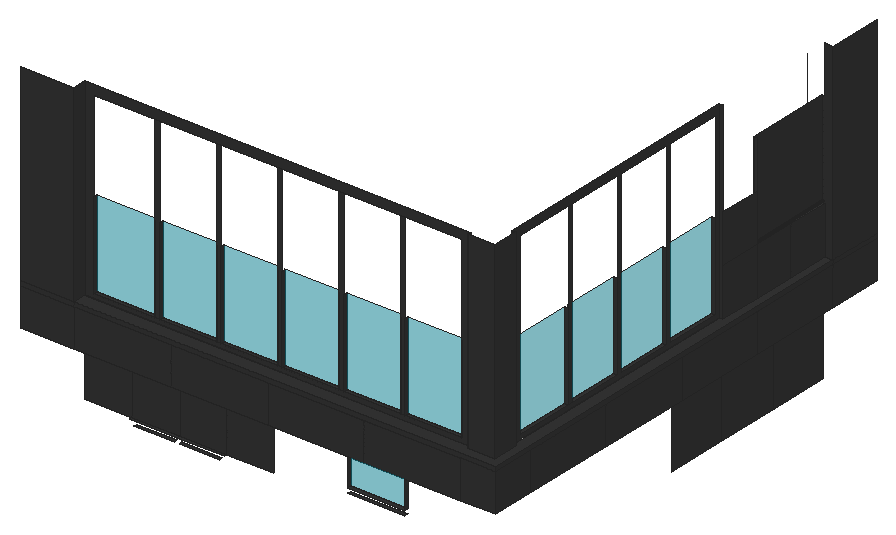
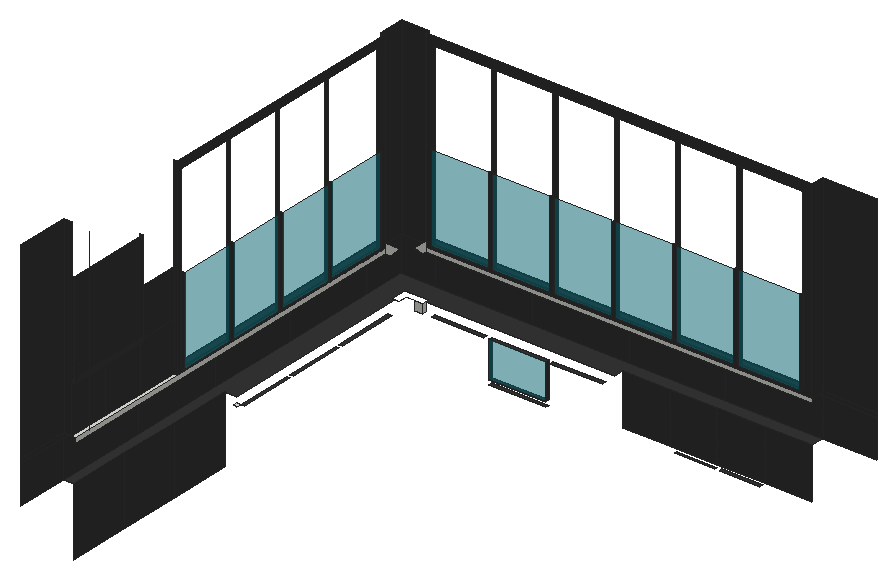
# SketchUp Ruby script. Lengths in inches.
U = 1.inch
M = Sketchup.active_model
def pt(a) = Geom::Point3d.new(a.map { |v| v * U })
def face(e, loops, mat)
  f = e.add_face(loops[0].map { |a| pt(a) })
  loops[1..].each { |l| e.add_face(l.map { |a| pt(a) }).erase! }
  f.material = f.back_material = mat if mat
  f
end
# faces: each face lists its corners as indices into pts; further lists are holes
def faces(e, pts, list, mat = nil) = list.each { |f| face(e, (f[0].is_a?(Array) ? f : [f]).map { |l| l.map { |i| pts[i] } }, mat) }
# xy, xz, yz: faces in a plane at the given z, y or x. An outline is a flat list of corners, or four numbers for a rectangle; further outlines are holes
def ring(l) = l.size == 4 ? [[l[0], l[1]], [l[2], l[1]], [l[2], l[3]], [l[0], l[3]]] : l.each_slice(2).to_a
def flat(e, list, mat, &to3) = list.each { |f| face(e, (f[0].is_a?(Array) ? f : [f]).map { |l| ring(l).map { |u, v| to3.(u, v) } }, mat) }
def xy(e, z, list, mat = nil) = flat(e, list, mat) { |x, y| [x, y, z] }
def xz(e, y, list, mat = nil) = flat(e, list, mat) { |x, z| [x, y, z] }
def yz(e, x, list, mat = nil) = flat(e, list, mat) { |y, z| [x, y, z] }
def lines(e, pts, list) = list.each { |a, b| e.add_line(pt(pts[a]), pt(pts[b])) }
# prism: a flat outline (further loops are holes) pulled along v
def prism(e, loops, v, mat = nil)
  f = face(e, loops, mat); d = Geom::Vector3d.new(v.map { |x| x * U })
  f.pushpull(f.normal.samedirection?(d) ? d.length : -d.length)
end
def box(e, o, s, mat = nil) = prism(e, [[o, [o[0] + s[0], o[1], o[2]], [o[0] + s[0], o[1] + s[1], o[2]], [o[0], o[1] + s[1], o[2]]]], [0, 0, s[2]], mat)
def at(x, y, z, deg = 0) = Geom::Transformation.translation(pt([x, y, z])) * Geom::Transformation.rotation(ORIGIN, Z_AXIS, deg.degrees)
def axes(o, x, y, z) = Geom::Transformation.new([*x, 0, *y, 0, *z, 0, *pt(o).to_a, 1])
def part(name) = M.definitions.add(name)
# library, detail: a bought-in or finely detailed component or shape, given as its bounding box
def library(name, o, s) = part(name).tap { |d| box(d.entities, o, s) }
def detail(e, o, s) = box(e.add_group.entities, o, s)
def put(e, d, t, mat = nil) = e.add_instance(d, t).tap { |i| i.material = mat if mat }
def group(e, t, mat = nil) = e.add_group.tap { |g| g.transformation = t; g.material = mat if mat }.entities
root = M.entities
M.materials.add("[0135_DarkGray]1").color = [53, 53, 53]
M.materials.add("[Translucent Glass Blue]1").color = [1, 149, 171]
M.materials["[Translucent Glass Blue]1"].alpha = 0.5
xy(root,197.67,[[554.94,728.6875,609.19,732.6875],[615.19,728.6875,669.44,732.6875]],"[0135_DarkGray]1")
xy(root,203.67,[[548.94,728.6875,612.19,732.6875],[612.19,728.6875,675.44,732.6875]],"[0135_DarkGray]1")
xy(root,204.96,[[827.03,745.6875,903.36,750.6875]],"[0135_DarkGray]1")
xy(root,211.2,[[827.03,745.6875,903.36,750.6875]],"[0135_DarkGray]1")
xy(root,259.5625,[[1018.69,1020.6875,1023.69,1026.6875]])
xy(root,259.5625,[[750.69,745.6875,821.03,750.6875],[827.03,745.6875,903.36,750.6875],[909.36,745.6875,979.69,750.6875],[1013.69,774.6875,1018.69,856.6875],[1013.69,862.6875,1018.69,938.6875],
  [1013.69,944.6875,1018.69,1020.6875]],"[0135_DarkGray]1")
xy(root,271.5625,[[485.69,714.6875,485.69,732.6875,738.69,732.6875,738.69,745.6875,991.69,745.6875,991.69,740.6875,1023.69,740.6875,1023.69,762.6875,1018.69,762.6875,1018.69,1026.6875,1035.69,1026.6875,1035.69,1278.6875,1049.69,1278.6875,1049.69,714.6875]],"[0135_DarkGray]1")
xy(root,328.25,[[1033.13,1108.6875,1038.13,1278.6875]])
xy(root,328.25,[[485.69,714.6875,1049.69,714.6875,1049.69,1278.6875,1038.13,1278.6875,1038.13,1108.6875,1033.13,1108.6875,1033.13,762.6875,1038.13,762.6875,1038.13,727.5625,1001.69,727.5625,1001.69,732.5625,485.69,732.5625]],"[0135_DarkGray]1")
xy(root,334.25,[[497.69,732.5625,579.69,737.5625],[585.69,732.5625,661.69,737.5625],[667.69,732.5625,743.69,737.5625],[749.69,732.5625,825.69,737.5625],[831.69,732.5625,907.69,737.5625],
  [913.69,732.5625,989.69,737.5625],[1028.13,774.6875,1033.13,856.6875],[1028.13,862.6875,1033.13,938.6875],[1028.13,944.6875,1033.13,1020.6875],[1028.13,1026.6875,1033.13,1102.6875]],"[0135_DarkGray]1")
xy(root,392.3125,[[1034.13,1165.35,1038.13,1222.02],[1034.13,1222.02,1038.13,1278.6875]],"[0135_DarkGray]1")
xy(root,393.26,[[1035.97,1165.35,1036.3125,1278.6875]],"[0135_DarkGray]1")
xy(root,395.86,[[1035.96,1165.35,1036.3,1278.6875]],"[0135_DarkGray]1")
xz(root,714.6875,[[413.69,271.5625,485.69,322.25],[485.69,271.5625,615.01,322.25],[615.01,271.5625,744.32,322.25],[744.32,271.5625,873.63,322.25],[873.63,271.5625,1002.94,322.25],
  [1002.94,271.5625,1049.69,322.25],[413.69,322.25,485.69,328.25],[485.69,322.25,1049.69,328.25],[413.69,328.25,485.69,584.5]],"[0135_DarkGray]1")
xz(root,727.5625,[[1001.69,328.25,1038.13,584.5]],"[0135_DarkGray]1")
xz(root,732.5625,[[485.69,322.25,1001.69,328.25]])
xz(root,732.5625,[[[485.69,328.25,1001.69,584.5],[497.69,334.25,989.69,572.5]],[579.69,334.25,585.69,572.5],[661.69,334.25,667.69,572.5],[743.69,334.25,749.69,572.5],[825.69,334.25,831.69,572.5],
  [907.69,334.25,913.69,572.5]],"[0135_DarkGray]1")
xz(root,732.6875,[[485.69,203.67,548.94,271.5625],[548.94,203.67,612.19,271.5625],[612.19,203.67,675.44,271.5625],[675.44,203.67,738.69,271.5625]],"[0135_DarkGray]1")
xz(root,737.5625,[[497.69,334.25,579.69,450.375],[585.69,334.25,661.69,450.375],[667.69,334.25,743.69,450.375],[749.69,334.25,825.69,450.375],[831.69,334.25,907.69,450.375],
  [913.69,334.25,989.69,450.375]],"[Translucent Glass Blue]1")
xz(root,750.6875,[[991.69,259.5625,1001.69,271.5625]])
xz(root,750.6875,[[827.03,211.2,903.36,259.5625]],"[Translucent Glass Blue]1")
xz(root,762.6875,[[1025.13,322.25,1033.13,322.25,1033.13,334.25,1013.69,334.25]])
xz(root,762.6875,[[1033.13,328.25,1038.13,584.5]],"[0135_DarkGray]1")
xz(root,774.6875,[[1028.13,334.25,1033.13,450.375]],"[0135_DarkGray]1")
xz(root,856.6875,[[1028.13,334.25,1033.13,450.375]],"[0135_DarkGray]1")
xz(root,862.6875,[[1028.13,334.25,1033.13,450.375]],"[0135_DarkGray]1")
xz(root,938.6875,[[1028.13,334.25,1033.13,450.375]],"[0135_DarkGray]1")
xz(root,944.6875,[[1028.13,334.25,1033.13,450.375]],"[0135_DarkGray]1")
xz(root,1020.6875,[[1028.13,334.25,1033.13,450.375]],"[0135_DarkGray]1")
xz(root,1026.6875,[[1028.13,334.25,1033.13,450.375]],"[0135_DarkGray]1")
xz(root,1102.6875,[[1028.13,334.25,1033.13,450.375]],"[0135_DarkGray]1")
xz(root,1108.6875,[[1033.13,328.25,1038.13,584.5]],"[0135_DarkGray]1")
xz(root,1165.35,[[[1034.13,392.3125,1038.13,520.4375],[1035.97,517.26,1036.3125,517.26,1036.64,517.35,1036.94,517.52,1037.18,517.77,1037.35,518.0625,1037.4375,518.4,1037.44,518.74,1037.34,519.07,1037.17,519.36,1036.93,519.61,1036.63,519.77,1036.3,519.86,1035.96,519.86,1035.625,519.77,1035.33,519.6,1035.09,519.35,1034.92,519.05,1034.83,518.72,1034.83,518.38,1034.93,518.05,1035.1,517.75,1035.34,517.51,1035.64,517.34],[1035.97,513.125,1036.3125,513.125,1036.64,513.22,1036.94,513.39,1037.18,513.63,1037.35,513.93,1037.4375,514.26,1037.44,514.6,1037.34,514.94,1037.17,515.23,1036.93,515.47,1036.63,515.64,1036.3,515.73,1035.96,515.73,1035.625,515.64,1035.33,515.46,1035.09,515.22,1034.92,514.92,1034.83,514.59,1034.83,514.25,1034.93,513.92,1035.1,513.62,1035.34,513.38,1035.64,513.21],[1035.97,508.99,1036.3125,508.99,1036.64,509.08,1036.94,509.26,1037.18,509.5,1037.35,509.8,1037.4375,510.13,1037.44,510.47,1037.34,510.8,1037.17,511.1,1036.93,511.34,1036.63,511.51,1036.3,511.6,1035.96,511.59,1035.625,511.5,1035.33,511.33,1035.09,511.09,1034.92,510.79,1034.83,510.46,1034.83,510.11,1034.93,509.78,1035.1,509.49,1035.34,509.25,1035.64,509.08],[1035.97,504.86,1036.3125,504.86,1036.64,504.95,1036.94,505.12,1037.18,505.37,1037.35,505.66,1037.4375,506,1037.44,506.34,1037.34,506.67,1037.17,506.96,1036.93,507.21,1036.63,507.375,1036.3,507.46,1035.96,507.46,1035.625,507.37,1035.33,507.2,1035.09,506.95,1034.92,506.65,1034.83,506.32,1034.83,505.98,1034.93,505.65,1035.1,505.35,1035.34,505.11,1035.64,504.94],[1035.97,500.72,1036.3125,500.73,1036.64,500.82,1036.94,500.99,1037.18,501.23,1037.35,501.53,1037.4375,501.86,1037.44,502.2,1037.34,502.54,1037.17,502.83,1036.93,503.07,1036.63,503.24,1036.3,503.33,1035.96,503.33,1035.625,503.24,1035.33,503.0625,1035.09,502.82,1034.92,502.52,1034.83,502.19,1034.83,501.85,1034.93,501.52,1035.1,501.22,1035.34,500.98,1035.64,500.8125],[1035.97,496.59,1036.3125,496.59,1036.64,496.68,1036.94,496.86,1037.18,497.1,1037.35,497.4,1037.4375,497.73,1037.44,498.07,1037.34,498.4,1037.17,498.7,1036.93,498.9375,1036.63,499.11,1036.3,499.2,1035.96,499.19,1035.625,499.1,1035.33,498.93,1035.09,498.6875,1034.92,498.39,1034.83,498.06,1034.83,497.71,1034.93,497.38,1035.1,497.09,1035.34,496.85,1035.64,496.68],[1035.97,492.46,1036.3125,492.46,1036.64,492.55,1036.94,492.72,1037.18,492.97,1037.35,493.26,1037.4375,493.6,1037.44,493.9375,1037.34,494.27,1037.17,494.5625,1036.93,494.81,1036.63,494.97,1036.3,495.0625,1035.96,495.06,1035.625,494.97,1035.33,494.8,1035.09,494.55,1034.92,494.25,1034.83,493.92,1034.83,493.58,1034.93,493.25,1035.1,492.95,1035.34,492.71,1035.64,492.54],[1035.97,488.32,1036.3125,488.33,1036.64,488.42,1036.94,488.59,1037.18,488.83,1037.35,489.13,1037.4375,489.46,1037.44,489.8,1037.34,490.14,1037.17,490.43,1036.93,490.67,1036.63,490.84,1036.3,490.93,1035.96,490.93,1035.625,490.84,1035.33,490.66,1035.09,490.42,1034.92,490.12,1034.83,489.79,1034.83,489.45,1034.93,489.12,1035.1,488.82,1035.34,488.58,1035.64,488.41],[1035.97,484.19,1036.3125,484.19,1036.64,484.28,1036.94,484.46,1037.18,484.7,1037.35,485,1037.4375,485.33,1037.44,485.67,1037.34,486,1037.17,486.3,1036.93,486.54,1036.63,486.71,1036.3,486.8,1035.96,486.79,1035.625,486.7,1035.33,486.53,1035.09,486.29,1034.92,485.99,1034.83,485.66,1034.83,485.3125,1034.93,484.98,1035.1,484.6875,1035.34,484.45,1035.64,484.28],[1035.97,480.06,1036.3125,480.06,1036.64,480.15,1036.94,480.32,1037.18,480.57,1037.35,480.86,1037.4375,481.2,1037.44,481.54,1037.34,481.87,1037.17,482.16,1036.93,482.41,1036.63,482.57,1036.3,482.66,1035.96,482.66,1035.625,482.57,1035.33,482.4,1035.09,482.15,1034.92,481.85,1034.83,481.52,1034.83,481.18,1034.93,480.85,1035.1,480.55,1035.34,480.3125,1035.64,480.14],[1035.97,475.92,1036.3125,475.93,1036.64,476.02,1036.94,476.1875,1037.18,476.43,1037.35,476.73,1037.4375,477.0625,1037.44,477.4,1037.34,477.74,1037.17,478.03,1036.93,478.27,1036.63,478.44,1036.3,478.53,1035.96,478.53,1035.625,478.4375,1035.33,478.26,1035.09,478.02,1034.92,477.72,1034.83,477.39,1034.83,477.05,1034.93,476.72,1035.1,476.42,1035.34,476.18,1035.64,476.01],[1035.97,471.79,1036.3125,471.79,1036.64,471.88,1036.94,472.06,1037.18,472.3,1037.35,472.6,1037.4375,472.93,1037.44,473.27,1037.34,473.6,1037.17,473.9,1036.93,474.14,1036.63,474.31,1036.3,474.4,1035.96,474.39,1035.625,474.3,1035.33,474.13,1035.09,473.89,1034.92,473.59,1034.83,473.26,1034.83,472.91,1034.93,472.58,1035.1,472.29,1035.34,472.05,1035.64,471.88],[1035.97,467.66,1036.3125,467.66,1036.64,467.75,1036.94,467.92,1037.18,468.17,1037.35,468.46,1037.4375,468.8,1037.44,469.14,1037.34,469.47,1037.17,469.76,1036.93,470.01,1036.63,470.17,1036.3,470.26,1035.96,470.26,1035.625,470.17,1035.33,470,1035.09,469.75,1034.92,469.45,1034.83,469.125,1034.83,468.78,1034.93,468.45,1035.1,468.15,1035.34,467.91,1035.64,467.74],[1035.97,463.52,1036.3125,463.53,1036.64,463.62,1036.94,463.79,1037.18,464.03,1037.35,464.33,1037.4375,464.66,1037.44,465,1037.34,465.34,1037.17,465.63,1036.93,465.87,1036.63,466.04,1036.3,466.13,1035.96,466.125,1035.625,466.04,1035.33,465.86,1035.09,465.62,1034.92,465.32,1034.83,464.99,1034.83,464.65,1034.93,464.32,1035.1,464.02,1035.34,463.78,1035.64,463.61],[1035.97,459.39,1036.3125,459.39,1036.64,459.48,1036.94,459.66,1037.18,459.9,1037.35,460.2,1037.4375,460.53,1037.44,460.87,1037.34,461.2,1037.17,461.5,1036.93,461.74,1036.63,461.91,1036.3,462,1035.96,461.99,1035.625,461.9,1035.33,461.73,1035.09,461.49,1034.92,461.1875,1034.83,460.86,1034.83,460.51,1034.93,460.18,1035.1,459.89,1035.34,459.65,1035.64,459.48],[1035.97,455.26,1036.3125,455.26,1036.64,455.35,1036.94,455.52,1037.18,455.77,1037.35,456.0625,1037.4375,456.4,1037.44,456.74,1037.34,457.07,1037.17,457.36,1036.93,457.61,1036.63,457.77,1036.3,457.86,1035.96,457.86,1035.625,457.77,1035.33,457.6,1035.09,457.35,1034.92,457.05,1034.83,456.72,1034.83,456.38,1034.93,456.05,1035.1,455.75,1035.34,455.51,1035.64,455.34],[1035.97,451.125,1036.3125,451.125,1036.64,451.22,1036.94,451.39,1037.18,451.63,1037.35,451.93,1037.4375,452.26,1037.44,452.6,1037.34,452.94,1037.17,453.23,1036.93,453.47,1036.63,453.64,1036.3,453.73,1035.96,453.73,1035.625,453.64,1035.33,453.46,1035.09,453.22,1034.92,452.92,1034.83,452.59,1034.83,452.25,1034.93,451.92,1035.1,451.62,1035.34,451.38,1035.64,451.21],[1035.97,446.99,1036.3125,446.99,1036.64,447.08,1036.94,447.26,1037.18,447.5,1037.35,447.8,1037.4375,448.13,1037.44,448.47,1037.34,448.8,1037.17,449.1,1036.93,449.34,1036.63,449.51,1036.3,449.6,1035.96,449.59,1035.625,449.5,1035.33,449.33,1035.09,449.09,1034.92,448.79,1034.83,448.46,1034.83,448.11,1034.93,447.78,1035.1,447.49,1035.34,447.25,1035.64,447.08],[1035.97,442.86,1036.3125,442.86,1036.64,442.95,1036.94,443.12,1037.18,443.37,1037.35,443.66,1037.4375,444,1037.44,444.34,1037.34,444.67,1037.17,444.96,1036.93,445.21,1036.63,445.375,1036.3,445.46,1035.96,445.46,1035.625,445.37,1035.33,445.2,1035.09,444.95,1034.92,444.65,1034.83,444.32,1034.83,443.98,1034.93,443.65,1035.1,443.35,1035.34,443.11,1035.64,442.94],[1035.97,438.72,1036.3125,438.73,1036.64,438.82,1036.94,438.99,1037.18,439.23,1037.35,439.53,1037.4375,439.86,1037.44,440.2,1037.34,440.54,1037.17,440.83,1036.93,441.07,1036.63,441.24,1036.3,441.33,1035.96,441.33,1035.625,441.24,1035.33,441.0625,1035.09,440.82,1034.92,440.52,1034.83,440.19,1034.83,439.85,1034.93,439.52,1035.1,439.22,1035.34,438.98,1035.64,438.8125],[1035.97,434.59,1036.3125,434.59,1036.64,434.68,1036.94,434.86,1037.18,435.1,1037.35,435.4,1037.4375,435.73,1037.44,436.07,1037.34,436.4,1037.17,436.7,1036.93,436.9375,1036.63,437.11,1036.3,437.2,1035.96,437.19,1035.625,437.1,1035.33,436.93,1035.09,436.6875,1034.92,436.39,1034.83,436.06,1034.83,435.71,1034.93,435.38,1035.1,435.09,1035.34,434.85,1035.64,434.68],[1035.97,430.46,1036.3125,430.46,1036.64,430.55,1036.94,430.72,1037.18,430.97,1037.35,431.26,1037.4375,431.6,1037.44,431.9375,1037.34,432.27,1037.17,432.5625,1036.93,432.81,1036.63,432.97,1036.3,433.0625,1035.96,433.06,1035.625,432.97,1035.33,432.8,1035.09,432.55,1034.92,432.25,1034.83,431.92,1034.83,431.58,1034.93,431.25,1035.1,430.95,1035.34,430.71,1035.64,430.54],[1035.97,426.32,1036.3125,426.33,1036.64,426.42,1036.94,426.59,1037.18,426.83,1037.35,427.13,1037.4375,427.46,1037.44,427.8,1037.34,428.14,1037.17,428.43,1036.93,428.67,1036.63,428.84,1036.3,428.93,1035.96,428.93,1035.625,428.84,1035.33,428.66,1035.09,428.42,1034.92,428.12,1034.83,427.79,1034.83,427.45,1034.93,427.12,1035.1,426.82,1035.34,426.58,1035.64,426.41],[1035.97,422.19,1036.3125,422.19,1036.64,422.28,1036.94,422.46,1037.18,422.7,1037.35,423,1037.4375,423.33,1037.44,423.67,1037.34,424,1037.17,424.3,1036.93,424.54,1036.63,424.71,1036.3,424.8,1035.96,424.79,1035.625,424.7,1035.33,424.53,1035.09,424.29,1034.92,423.99,1034.83,423.66,1034.83,423.3125,1034.93,422.98,1035.1,422.6875,1035.34,422.45,1035.64,422.28],[1035.97,418.06,1036.3125,418.06,1036.64,418.15,1036.94,418.32,1037.18,418.57,1037.35,418.86,1037.4375,419.2,1037.44,419.54,1037.34,419.87,1037.17,420.16,1036.93,420.41,1036.63,420.57,1036.3,420.66,1035.96,420.66,1035.625,420.57,1035.33,420.4,1035.09,420.15,1034.92,419.85,1034.83,419.52,1034.83,419.18,1034.93,418.85,1035.1,418.55,1035.34,418.3125,1035.64,418.14],[1035.97,413.92,1036.3125,413.93,1036.64,414.02,1036.94,414.1875,1037.18,414.43,1037.35,414.73,1037.4375,415.0625,1037.44,415.4,1037.34,415.74,1037.17,416.03,1036.93,416.27,1036.63,416.44,1036.3,416.53,1035.96,416.53,1035.625,416.4375,1035.33,416.26,1035.09,416.02,1034.92,415.72,1034.83,415.39,1034.83,415.05,1034.93,414.72,1035.1,414.42,1035.34,414.18,1035.64,414.01],[1035.97,409.79,1036.3125,409.79,1036.64,409.88,1036.94,410.06,1037.18,410.3,1037.35,410.6,1037.4375,410.93,1037.44,411.27,1037.34,411.6,1037.17,411.9,1036.93,412.14,1036.63,412.31,1036.3,412.4,1035.96,412.39,1035.625,412.3,1035.33,412.13,1035.09,411.89,1034.92,411.59,1034.83,411.26,1034.83,410.91,1034.93,410.58,1035.1,410.29,1035.34,410.05,1035.64,409.88],[1035.97,405.66,1036.3125,405.66,1036.64,405.75,1036.94,405.92,1037.18,406.17,1037.35,406.46,1037.4375,406.8,1037.44,407.14,1037.34,407.47,1037.17,407.76,1036.93,408.01,1036.63,408.17,1036.3,408.26,1035.96,408.26,1035.625,408.17,1035.33,408,1035.09,407.75,1034.92,407.45,1034.83,407.125,1034.83,406.78,1034.93,406.45,1035.1,406.15,1035.34,405.91,1035.64,405.74],[1035.97,401.52,1036.3125,401.53,1036.64,401.62,1036.94,401.79,1037.18,402.03,1037.35,402.33,1037.4375,402.66,1037.44,403,1037.34,403.34,1037.17,403.63,1036.93,403.87,1036.63,404.04,1036.3,404.13,1035.96,404.125,1035.625,404.04,1035.33,403.86,1035.09,403.62,1034.92,403.32,1034.83,402.99,1034.83,402.65,1034.93,402.32,1035.1,402.02,1035.34,401.78,1035.64,401.61],[1035.97,397.39,1036.3125,397.39,1036.64,397.48,1036.94,397.66,1037.18,397.9,1037.35,398.2,1037.4375,398.53,1037.44,398.87,1037.34,399.2,1037.17,399.5,1036.93,399.74,1036.63,399.91,1036.3,400,1035.96,399.99,1035.625,399.9,1035.33,399.73,1035.09,399.49,1034.92,399.1875,1034.83,398.86,1034.83,398.51,1034.93,398.18,1035.1,397.89,1035.34,397.65,1035.64,397.48],[1035.97,393.26,1036.3125,393.26,1036.64,393.35,1036.94,393.52,1037.18,393.77,1037.35,394.0625,1037.4375,394.4,1037.44,394.74,1037.34,395.07,1037.17,395.36,1036.93,395.61,1036.63,395.77,1036.3,395.86,1035.96,395.86,1035.625,395.77,1035.33,395.6,1035.09,395.35,1034.92,395.05,1034.83,394.72,1034.83,394.38,1034.93,394.05,1035.1,393.75,1035.34,393.51,1035.64,393.34]]],"[0135_DarkGray]1")
xz(root,1278.6875,[[[1038.13,328.25,1049.69,328.25,1049.69,584.5,1038.13,584.5,1038.13,520.4375,1034.13,520.4375,1034.13,392.3125,1038.13,392.3125],[1035.97,517.26,1035.64,517.34,1035.34,517.51,1035.1,517.75,1034.93,518.05,1034.83,518.38,1034.83,518.72,1034.92,519.05,1035.09,519.35,1035.33,519.6,1035.625,519.77,1035.96,519.86,1036.3,519.86,1036.63,519.77,1036.93,519.61,1037.17,519.36,1037.34,519.07,1037.44,518.74,1037.4375,518.4,1037.35,518.0625,1037.18,517.77,1036.94,517.52,1036.64,517.35,1036.3125,517.26],[1035.97,513.125,1035.64,513.21,1035.34,513.38,1035.1,513.62,1034.93,513.92,1034.83,514.25,1034.83,514.59,1034.92,514.92,1035.09,515.22,1035.33,515.46,1035.625,515.64,1035.96,515.73,1036.3,515.73,1036.63,515.64,1036.93,515.47,1037.17,515.23,1037.34,514.94,1037.44,514.6,1037.4375,514.26,1037.35,513.93,1037.18,513.63,1036.94,513.39,1036.64,513.22,1036.3125,513.125],[1035.97,508.99,1035.64,509.08,1035.34,509.25,1035.1,509.49,1034.93,509.78,1034.83,510.11,1034.83,510.46,1034.92,510.79,1035.09,511.09,1035.33,511.33,1035.625,511.5,1035.96,511.59,1036.3,511.6,1036.63,511.51,1036.93,511.34,1037.17,511.1,1037.34,510.8,1037.44,510.47,1037.4375,510.13,1037.35,509.8,1037.18,509.5,1036.94,509.26,1036.64,509.08,1036.3125,508.99],[1035.97,504.86,1035.64,504.94,1035.34,505.11,1035.1,505.35,1034.93,505.65,1034.83,505.98,1034.83,506.32,1034.92,506.65,1035.09,506.95,1035.33,507.2,1035.625,507.37,1035.96,507.46,1036.3,507.46,1036.63,507.375,1036.93,507.21,1037.17,506.96,1037.34,506.67,1037.44,506.34,1037.4375,506,1037.35,505.66,1037.18,505.37,1036.94,505.12,1036.64,504.95,1036.3125,504.86],[1035.97,500.72,1035.64,500.8125,1035.34,500.98,1035.1,501.22,1034.93,501.52,1034.83,501.85,1034.83,502.19,1034.92,502.52,1035.09,502.82,1035.33,503.0625,1035.625,503.24,1035.96,503.33,1036.3,503.33,1036.63,503.24,1036.93,503.07,1037.17,502.83,1037.34,502.54,1037.44,502.2,1037.4375,501.86,1037.35,501.53,1037.18,501.23,1036.94,500.99,1036.64,500.82,1036.3125,500.73],[1035.97,496.59,1035.64,496.68,1035.34,496.85,1035.1,497.09,1034.93,497.38,1034.83,497.71,1034.83,498.06,1034.92,498.39,1035.09,498.6875,1035.33,498.93,1035.625,499.1,1035.96,499.19,1036.3,499.2,1036.63,499.11,1036.93,498.9375,1037.17,498.7,1037.34,498.4,1037.44,498.07,1037.4375,497.73,1037.35,497.4,1037.18,497.1,1036.94,496.86,1036.64,496.68,1036.3125,496.59],[1035.97,492.46,1035.64,492.54,1035.34,492.71,1035.1,492.95,1034.93,493.25,1034.83,493.58,1034.83,493.92,1034.92,494.25,1035.09,494.55,1035.33,494.8,1035.625,494.97,1035.96,495.06,1036.3,495.0625,1036.63,494.97,1036.93,494.81,1037.17,494.5625,1037.34,494.27,1037.44,493.9375,1037.4375,493.6,1037.35,493.26,1037.18,492.97,1036.94,492.72,1036.64,492.55,1036.3125,492.46],[1035.97,488.32,1035.64,488.41,1035.34,488.58,1035.1,488.82,1034.93,489.12,1034.83,489.45,1034.83,489.79,1034.92,490.12,1035.09,490.42,1035.33,490.66,1035.625,490.84,1035.96,490.93,1036.3,490.93,1036.63,490.84,1036.93,490.67,1037.17,490.43,1037.34,490.14,1037.44,489.8,1037.4375,489.46,1037.35,489.13,1037.18,488.83,1036.94,488.59,1036.64,488.42,1036.3125,488.33],[1035.97,484.19,1035.64,484.28,1035.34,484.45,1035.1,484.6875,1034.93,484.98,1034.83,485.3125,1034.83,485.66,1034.92,485.99,1035.09,486.29,1035.33,486.53,1035.625,486.7,1035.96,486.79,1036.3,486.8,1036.63,486.71,1036.93,486.54,1037.17,486.3,1037.34,486,1037.44,485.67,1037.4375,485.33,1037.35,485,1037.18,484.7,1036.94,484.46,1036.64,484.28,1036.3125,484.19],[1035.97,480.06,1035.64,480.14,1035.34,480.3125,1035.1,480.55,1034.93,480.85,1034.83,481.18,1034.83,481.52,1034.92,481.85,1035.09,482.15,1035.33,482.4,1035.625,482.57,1035.96,482.66,1036.3,482.66,1036.63,482.57,1036.93,482.41,1037.17,482.16,1037.34,481.87,1037.44,481.54,1037.4375,481.2,1037.35,480.86,1037.18,480.57,1036.94,480.32,1036.64,480.15,1036.3125,480.06],[1035.97,475.92,1035.64,476.01,1035.34,476.18,1035.1,476.42,1034.93,476.72,1034.83,477.05,1034.83,477.39,1034.92,477.72,1035.09,478.02,1035.33,478.26,1035.625,478.4375,1035.96,478.53,1036.3,478.53,1036.63,478.44,1036.93,478.27,1037.17,478.03,1037.34,477.74,1037.44,477.4,1037.4375,477.0625,1037.35,476.73,1037.18,476.43,1036.94,476.1875,1036.64,476.02,1036.3125,475.93],[1035.97,471.79,1035.64,471.88,1035.34,472.05,1035.1,472.29,1034.93,472.58,1034.83,472.91,1034.83,473.26,1034.92,473.59,1035.09,473.89,1035.33,474.13,1035.625,474.3,1035.96,474.39,1036.3,474.4,1036.63,474.31,1036.93,474.14,1037.17,473.9,1037.34,473.6,1037.44,473.27,1037.4375,472.93,1037.35,472.6,1037.18,472.3,1036.94,472.06,1036.64,471.88,1036.3125,471.79],[1035.97,467.66,1035.64,467.74,1035.34,467.91,1035.1,468.15,1034.93,468.45,1034.83,468.78,1034.83,469.125,1034.92,469.45,1035.09,469.75,1035.33,470,1035.625,470.17,1035.96,470.26,1036.3,470.26,1036.63,470.17,1036.93,470.01,1037.17,469.76,1037.34,469.47,1037.44,469.14,1037.4375,468.8,1037.35,468.46,1037.18,468.17,1036.94,467.92,1036.64,467.75,1036.3125,467.66],[1035.97,463.52,1035.64,463.61,1035.34,463.78,1035.1,464.02,1034.93,464.32,1034.83,464.65,1034.83,464.99,1034.92,465.32,1035.09,465.62,1035.33,465.86,1035.625,466.04,1035.96,466.125,1036.3,466.13,1036.63,466.04,1036.93,465.87,1037.17,465.63,1037.34,465.34,1037.44,465,1037.4375,464.66,1037.35,464.33,1037.18,464.03,1036.94,463.79,1036.64,463.62,1036.3125,463.53],[1035.97,459.39,1035.64,459.48,1035.34,459.65,1035.1,459.89,1034.93,460.18,1034.83,460.51,1034.83,460.86,1034.92,461.1875,1035.09,461.49,1035.33,461.73,1035.625,461.9,1035.96,461.99,1036.3,462,1036.63,461.91,1036.93,461.74,1037.17,461.5,1037.34,461.2,1037.44,460.87,1037.4375,460.53,1037.35,460.2,1037.18,459.9,1036.94,459.66,1036.64,459.48,1036.3125,459.39],[1035.97,455.26,1035.64,455.34,1035.34,455.51,1035.1,455.75,1034.93,456.05,1034.83,456.38,1034.83,456.72,1034.92,457.05,1035.09,457.35,1035.33,457.6,1035.625,457.77,1035.96,457.86,1036.3,457.86,1036.63,457.77,1036.93,457.61,1037.17,457.36,1037.34,457.07,1037.44,456.74,1037.4375,456.4,1037.35,456.0625,1037.18,455.77,1036.94,455.52,1036.64,455.35,1036.3125,455.26],[1035.97,451.125,1035.64,451.21,1035.34,451.38,1035.1,451.62,1034.93,451.92,1034.83,452.25,1034.83,452.59,1034.92,452.92,1035.09,453.22,1035.33,453.46,1035.625,453.64,1035.96,453.73,1036.3,453.73,1036.63,453.64,1036.93,453.47,1037.17,453.23,1037.34,452.94,1037.44,452.6,1037.4375,452.26,1037.35,451.93,1037.18,451.63,1036.94,451.39,1036.64,451.22,1036.3125,451.125],[1035.97,446.99,1035.64,447.08,1035.34,447.25,1035.1,447.49,1034.93,447.78,1034.83,448.11,1034.83,448.46,1034.92,448.79,1035.09,449.09,1035.33,449.33,1035.625,449.5,1035.96,449.59,1036.3,449.6,1036.63,449.51,1036.93,449.34,1037.17,449.1,1037.34,448.8,1037.44,448.47,1037.4375,448.13,1037.35,447.8,1037.18,447.5,1036.94,447.26,1036.64,447.08,1036.3125,446.99],[1035.97,442.86,1035.64,442.94,1035.34,443.11,1035.1,443.35,1034.93,443.65,1034.83,443.98,1034.83,444.32,1034.92,444.65,1035.09,444.95,1035.33,445.2,1035.625,445.37,1035.96,445.46,1036.3,445.46,1036.63,445.375,1036.93,445.21,1037.17,444.96,1037.34,444.67,1037.44,444.34,1037.4375,444,1037.35,443.66,1037.18,443.37,1036.94,443.12,1036.64,442.95,1036.3125,442.86],[1035.97,438.72,1035.64,438.8125,1035.34,438.98,1035.1,439.22,1034.93,439.52,1034.83,439.85,1034.83,440.19,1034.92,440.52,1035.09,440.82,1035.33,441.0625,1035.625,441.24,1035.96,441.33,1036.3,441.33,1036.63,441.24,1036.93,441.07,1037.17,440.83,1037.34,440.54,1037.44,440.2,1037.4375,439.86,1037.35,439.53,1037.18,439.23,1036.94,438.99,1036.64,438.82,1036.3125,438.73],[1035.97,434.59,1035.64,434.68,1035.34,434.85,1035.1,435.09,1034.93,435.38,1034.83,435.71,1034.83,436.06,1034.92,436.39,1035.09,436.6875,1035.33,436.93,1035.625,437.1,1035.96,437.19,1036.3,437.2,1036.63,437.11,1036.93,436.9375,1037.17,436.7,1037.34,436.4,1037.44,436.07,1037.4375,435.73,1037.35,435.4,1037.18,435.1,1036.94,434.86,1036.64,434.68,1036.3125,434.59],[1035.97,430.46,1035.64,430.54,1035.34,430.71,1035.1,430.95,1034.93,431.25,1034.83,431.58,1034.83,431.92,1034.92,432.25,1035.09,432.55,1035.33,432.8,1035.625,432.97,1035.96,433.06,1036.3,433.0625,1036.63,432.97,1036.93,432.81,1037.17,432.5625,1037.34,432.27,1037.44,431.9375,1037.4375,431.6,1037.35,431.26,1037.18,430.97,1036.94,430.72,1036.64,430.55,1036.3125,430.46],[1035.97,426.32,1035.64,426.41,1035.34,426.58,1035.1,426.82,1034.93,427.12,1034.83,427.45,1034.83,427.79,1034.92,428.12,1035.09,428.42,1035.33,428.66,1035.625,428.84,1035.96,428.93,1036.3,428.93,1036.63,428.84,1036.93,428.67,1037.17,428.43,1037.34,428.14,1037.44,427.8,1037.4375,427.46,1037.35,427.13,1037.18,426.83,1036.94,426.59,1036.64,426.42,1036.3125,426.33],[1035.97,422.19,1035.64,422.28,1035.34,422.45,1035.1,422.6875,1034.93,422.98,1034.83,423.3125,1034.83,423.66,1034.92,423.99,1035.09,424.29,1035.33,424.53,1035.625,424.7,1035.96,424.79,1036.3,424.8,1036.63,424.71,1036.93,424.54,1037.17,424.3,1037.34,424,1037.44,423.67,1037.4375,423.33,1037.35,423,1037.18,422.7,1036.94,422.46,1036.64,422.28,1036.3125,422.19],[1035.97,418.06,1035.64,418.14,1035.34,418.3125,1035.1,418.55,1034.93,418.85,1034.83,419.18,1034.83,419.52,1034.92,419.85,1035.09,420.15,1035.33,420.4,1035.625,420.57,1035.96,420.66,1036.3,420.66,1036.63,420.57,1036.93,420.41,1037.17,420.16,1037.34,419.87,1037.44,419.54,1037.4375,419.2,1037.35,418.86,1037.18,418.57,1036.94,418.32,1036.64,418.15,1036.3125,418.06],[1035.97,413.92,1035.64,414.01,1035.34,414.18,1035.1,414.42,1034.93,414.72,1034.83,415.05,1034.83,415.39,1034.92,415.72,1035.09,416.02,1035.33,416.26,1035.625,416.4375,1035.96,416.53,1036.3,416.53,1036.63,416.44,1036.93,416.27,1037.17,416.03,1037.34,415.74,1037.44,415.4,1037.4375,415.0625,1037.35,414.73,1037.18,414.43,1036.94,414.1875,1036.64,414.02,1036.3125,413.93],[1035.97,409.79,1035.64,409.88,1035.34,410.05,1035.1,410.29,1034.93,410.58,1034.83,410.91,1034.83,411.26,1034.92,411.59,1035.09,411.89,1035.33,412.13,1035.625,412.3,1035.96,412.39,1036.3,412.4,1036.63,412.31,1036.93,412.14,1037.17,411.9,1037.34,411.6,1037.44,411.27,1037.4375,410.93,1037.35,410.6,1037.18,410.3,1036.94,410.06,1036.64,409.88,1036.3125,409.79],[1035.97,405.66,1035.64,405.74,1035.34,405.91,1035.1,406.15,1034.93,406.45,1034.83,406.78,1034.83,407.125,1034.92,407.45,1035.09,407.75,1035.33,408,1035.625,408.17,1035.96,408.26,1036.3,408.26,1036.63,408.17,1036.93,408.01,1037.17,407.76,1037.34,407.47,1037.44,407.14,1037.4375,406.8,1037.35,406.46,1037.18,406.17,1036.94,405.92,1036.64,405.75,1036.3125,405.66],[1035.97,401.52,1035.64,401.61,1035.34,401.78,1035.1,402.02,1034.93,402.32,1034.83,402.65,1034.83,402.99,1034.92,403.32,1035.09,403.62,1035.33,403.86,1035.625,404.04,1035.96,404.125,1036.3,404.13,1036.63,404.04,1036.93,403.87,1037.17,403.63,1037.34,403.34,1037.44,403,1037.4375,402.66,1037.35,402.33,1037.18,402.03,1036.94,401.79,1036.64,401.62,1036.3125,401.53],[1035.97,397.39,1035.64,397.48,1035.34,397.65,1035.1,397.89,1034.93,398.18,1034.83,398.51,1034.83,398.86,1034.92,399.1875,1035.09,399.49,1035.33,399.73,1035.625,399.9,1035.96,399.99,1036.3,400,1036.63,399.91,1036.93,399.74,1037.17,399.5,1037.34,399.2,1037.44,398.87,1037.4375,398.53,1037.35,398.2,1037.18,397.9,1036.94,397.66,1036.64,397.48,1036.3125,397.39],[1035.97,393.26,1035.64,393.34,1035.34,393.51,1035.1,393.75,1034.93,394.05,1034.83,394.38,1034.83,394.72,1034.92,395.05,1035.09,395.35,1035.33,395.6,1035.625,395.77,1035.96,395.86,1036.3,395.86,1036.63,395.77,1036.93,395.61,1037.17,395.36,1037.34,395.07,1037.44,394.74,1037.4375,394.4,1037.35,394.0625,1037.18,393.77,1036.94,393.52,1036.64,393.35,1036.3125,393.26]]],"[0135_DarkGray]1")
yz(root,485.69,[[714.6875,328.25,732.5625,584.5]],"[0135_DarkGray]1")
yz(root,497.69,[[732.5625,334.25,737.5625,450.375]],"[0135_DarkGray]1")
yz(root,579.69,[[732.5625,334.25,737.5625,450.375]],"[0135_DarkGray]1")
yz(root,585.69,[[732.5625,334.25,737.5625,450.375]],"[0135_DarkGray]1")
yz(root,661.69,[[732.5625,334.25,737.5625,450.375]],"[0135_DarkGray]1")
yz(root,667.69,[[732.5625,334.25,737.5625,450.375]],"[0135_DarkGray]1")
yz(root,743.69,[[732.5625,334.25,737.5625,448.5]],"[0135_DarkGray]1")
yz(root,749.69,[[732.5625,334.25,737.5625,448.5]],"[0135_DarkGray]1")
yz(root,825.69,[[732.5625,334.25,737.5625,450.375]],"[0135_DarkGray]1")
yz(root,827.03,[[745.6875,211.2,750.6875,259.5625]],"[0135_DarkGray]1")
yz(root,831.69,[[732.5625,334.25,737.5625,450.375]],"[0135_DarkGray]1")
yz(root,903.36,[[745.6875,211.2,750.6875,259.5625]],"[0135_DarkGray]1")
yz(root,907.69,[[732.5625,334.25,737.5625,450.375]],"[0135_DarkGray]1")
yz(root,913.69,[[732.5625,334.25,737.5625,450.375]],"[0135_DarkGray]1")
yz(root,989.69,[[732.5625,334.25,737.5625,450.375]],"[0135_DarkGray]1")
yz(root,991.69,[[745.6875,259.5625,750.6875,271.5625]])
yz(root,1001.69,[[732.5625,322.25,732.5625,334.25,750.6875,334.25,737.5625,322.25]])
yz(root,1001.69,[[727.5625,328.25,732.5625,584.5]],"[0135_DarkGray]1")
yz(root,1028.13,[[774.6875,334.25,856.6875,450.375],[862.6875,334.25,938.6875,450.375],[944.6875,334.25,1020.6875,450.375],[1026.6875,334.25,1102.6875,450.375]],"[Translucent Glass Blue]1")
yz(root,1033.13,[[762.6875,322.25,1278.6875,328.25]])
yz(root,1033.13,[[762.6875,328.25,1108.6875,328.25,1108.6875,334.25,1026.6875,334.25,1026.6875,572.5,1020.6875,572.5,1020.6875,334.25,944.6875,334.25,944.6875,572.5,938.6875,572.5,938.6875,334.25,774.6875,334.25,774.6875,572.5,1102.6875,572.5,1102.6875,334.25,1108.6875,334.25,1108.6875,584.5,762.6875,584.5],[856.6875,334.25,862.6875,572.5]],"[0135_DarkGray]1")
yz(root,1034.13,[[1165.35,392.3125,1278.6875,520.4375]],"[0135_DarkGray]1")
yz(root,1034.83,[[1165.35,394.38,1278.6875,394.72]],"[0135_DarkGray]1")
yz(root,1035.69,[[1026.6875,181.04,1110.6875,271.5625],[1110.6875,181.04,1194.6875,271.5625],[1194.6875,181.04,1278.6875,271.5625]],"[0135_DarkGray]1")
yz(root,1038.13,[[727.5625,328.25,762.6875,584.5],[1108.6875,328.25,1165.35,392.3125],[1165.35,328.25,1222.02,392.3125],[1222.02,328.25,1278.6875,392.3125],[1108.6875,392.3125,1165.35,456.375]],"[0135_DarkGray]1")
yz(root,1049.69,[[714.6875,271.5625,771.9375,322.25],[771.9375,271.5625,898.625,322.25],[898.625,271.5625,1025.3125,322.25],[1025.3125,271.5625,1152,322.25],[1152,271.5625,1278.6875,322.25],
  [1278.6875,271.5625,1350.6875,322.25],[714.6875,322.25,1278.6875,328.25],[1278.6875,322.25,1350.6875,328.25],[1278.6875,328.25,1350.6875,584.5]],"[0135_DarkGray]1")
p = [[1035.64,1165.35,393.34],[1035.34,1165.35,393.51],[1035.34,1278.6875,393.51],[1035.64,1278.6875,393.34],[1035.97,1165.35,393.26],[1035.97,1278.6875,393.26],
  [1036.64,1165.35,393.35],[1036.3125,1165.35,393.26],[1036.3125,1278.6875,393.26],[1036.64,1278.6875,393.35],[1036.94,1165.35,393.52],[1036.94,1278.6875,393.52],
  [1035.1,1165.35,393.75],[1035.1,1278.6875,393.75],[1037.18,1165.35,393.77],[1037.18,1278.6875,393.77],[1034.93,1165.35,394.05],[1034.93,1278.6875,394.05],
  [1037.35,1165.35,394.0625],[1037.35,1278.6875,394.0625],[1034.83,1165.35,394.38],[1034.83,1278.6875,394.38],[1037.4375,1165.35,394.4],[1037.4375,1278.6875,394.4],
  [1037.44,1165.35,394.74],[1037.44,1278.6875,394.74],[1034.83,1165.35,394.72],[1034.92,1165.35,395.05],[1034.92,1278.6875,395.05],[1034.83,1278.6875,394.72],
  [1037.34,1165.35,395.07],[1037.34,1278.6875,395.07],[1035.09,1165.35,395.35],[1035.09,1278.6875,395.35],[1037.17,1165.35,395.36],[1037.17,1278.6875,395.36],
  [1035.33,1165.35,395.6],[1035.33,1278.6875,395.6],[1036.93,1165.35,395.61],[1036.93,1278.6875,395.61],[1035.625,1165.35,395.77],[1035.625,1278.6875,395.77],
  [1036.63,1165.35,395.77],[1036.63,1278.6875,395.77],[1035.96,1165.35,395.86],[1035.96,1278.6875,395.86],[1036.3,1165.35,395.86],[1036.3,1278.6875,395.86],
  [1013.69,750.6875,271.5625],[1013.69,762.6875,271.5625],[1025.13,1266.6875,334.25],[1025.13,1266.6875,572.5],[1001.69,750.6875,271.5625],[1018.69,762.6875,271.5625]]
faces(root,p,[[0,1,2,3],[4,0,3,5],[6,7,8,9],[10,6,9,11],[1,12,13,2],[14,10,11,15],[12,16,17,13],[18,14,15,19],
  [16,20,21,17],[22,18,19,23],[24,22,23,25],[26,27,28,29],[30,24,25,31],[27,32,33,28],[34,30,31,35],[32,36,37,33],
  [38,34,35,39],[36,40,41,37],[42,38,39,43],[40,44,45,41],[46,42,43,47]],"[0135_DarkGray]1")
lines(root,p,[[48,49],[50,51],[52,48],[49,53]])
